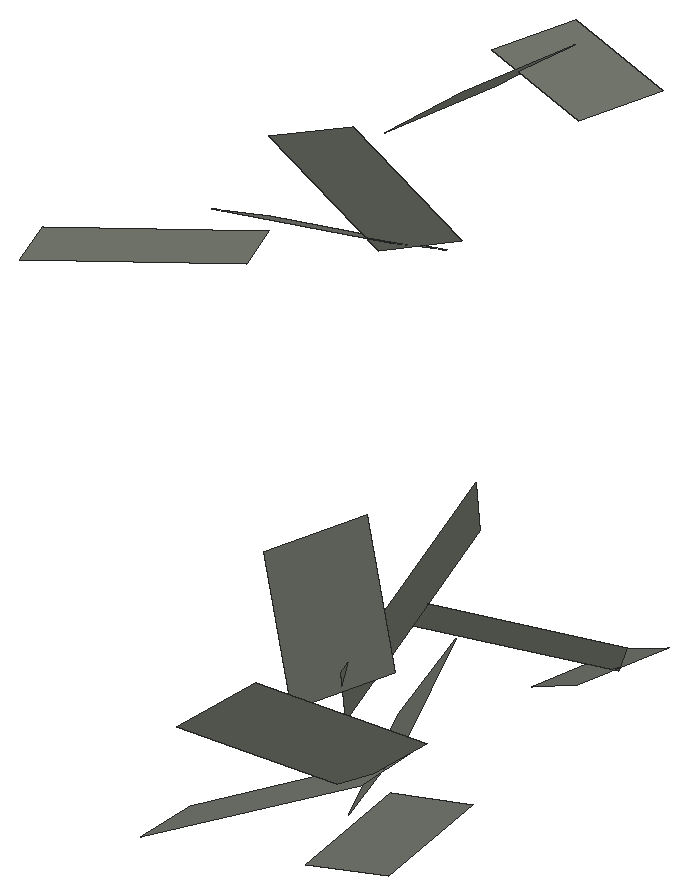
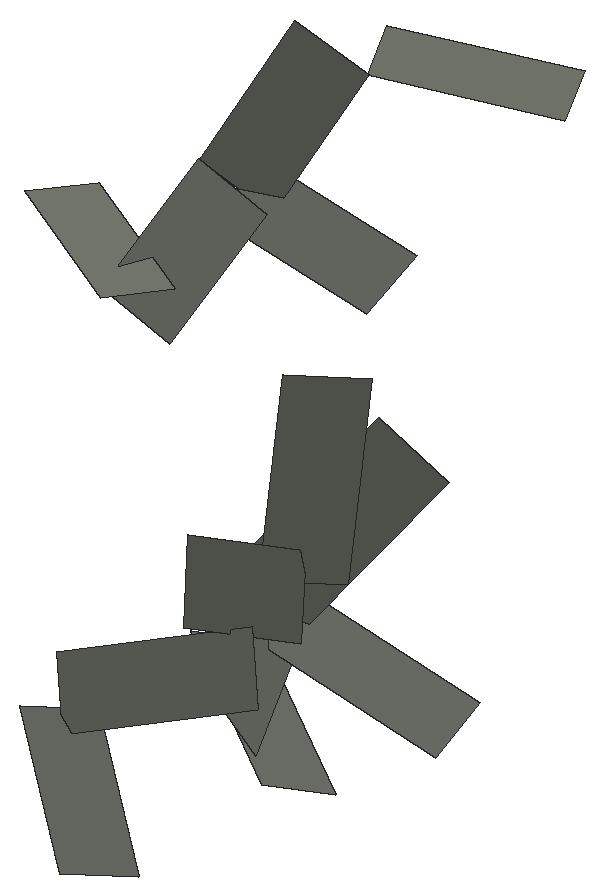
# SketchUp Ruby script. Lengths in inches.
U = 1.inch
M = Sketchup.active_model
def pt(a) = Geom::Point3d.new(a.map { |v| v * U })
def face(e, loops, mat)
  f = e.add_face(loops[0].map { |a| pt(a) })
  loops[1..].each { |l| e.add_face(l.map { |a| pt(a) }).erase! }
  f.material = f.back_material = mat if mat
  f
end
# faces: each face lists its corners as indices into pts; further lists are holes
def faces(e, pts, list, mat = nil) = list.each { |f| face(e, (f[0].is_a?(Array) ? f : [f]).map { |l| l.map { |i| pts[i] } }, mat) }
# xy, xz, yz: faces in a plane at the given z, y or x. An outline is a flat list of corners, or four numbers for a rectangle; further outlines are holes
def ring(l) = l.size == 4 ? [[l[0], l[1]], [l[2], l[1]], [l[2], l[3]], [l[0], l[3]]] : l.each_slice(2).to_a
def flat(e, list, mat, &to3) = list.each { |f| face(e, (f[0].is_a?(Array) ? f : [f]).map { |l| ring(l).map { |u, v| to3.(u, v) } }, mat) }
def xy(e, z, list, mat = nil) = flat(e, list, mat) { |x, y| [x, y, z] }
def xz(e, y, list, mat = nil) = flat(e, list, mat) { |x, z| [x, y, z] }
def yz(e, x, list, mat = nil) = flat(e, list, mat) { |y, z| [x, y, z] }
def lines(e, pts, list) = list.each { |a, b| e.add_line(pt(pts[a]), pt(pts[b])) }
# prism: a flat outline (further loops are holes) pulled along v
def prism(e, loops, v, mat = nil)
  f = face(e, loops, mat); d = Geom::Vector3d.new(v.map { |x| x * U })
  f.pushpull(f.normal.samedirection?(d) ? d.length : -d.length)
end
def box(e, o, s, mat = nil) = prism(e, [[o, [o[0] + s[0], o[1], o[2]], [o[0] + s[0], o[1] + s[1], o[2]], [o[0], o[1] + s[1], o[2]]]], [0, 0, s[2]], mat)
def at(x, y, z, deg = 0) = Geom::Transformation.translation(pt([x, y, z])) * Geom::Transformation.rotation(ORIGIN, Z_AXIS, deg.degrees)
def axes(o, x, y, z) = Geom::Transformation.new([*x, 0, *y, 0, *z, 0, *pt(o).to_a, 1])
def part(name) = M.definitions.add(name)
# library, detail: a bought-in or finely detailed component or shape, given as its bounding box
def library(name, o, s) = part(name).tap { |d| box(d.entities, o, s) }
def detail(e, o, s) = box(e.add_group.entities, o, s)
def put(e, d, t, mat = nil) = e.add_instance(d, t).tap { |i| i.material = mat if mat }
def group(e, t, mat = nil) = e.add_group.tap { |g| g.transformation = t; g.material = mat if mat }.entities
root = M.entities
M.materials.add("viburnumbladsadfasdfad0w122").color = [125, 129, 119]
c1 = part("Component\#315")
p = [[0.25,0,0],[2.05,0.01,0.35],[1.81,4.2,1.66],[0,4.19,1.3125]]
faces(c1.entities,p,[[0,1,2,3]],"viburnumbladsadfasdfad0w122")
c2 = part("viburnumblad2")
put(c2.entities,c1,axes([-19.23,-4.49,-32.18],[83.35428,0,0],[0,79.38502,0],[0,0,83.35428]))
put(root,c2,axes([2192.125,265.73,30.04],[-0.00355,0.00962,-0.00319],[-0.00963,-0.00512,-0.00451],[-0.00533,0.00188,0.0087]))
put(root,c2,axes([2192.16,269.91,28.65],[0.00165,0.00828,-0.00613],[-0.01063,-0.00165,-0.00484],[-0.00434,0.00735,0.00651]))
put(root,c2,axes([2192.3,268.57,18.41],[-0.00076,0.01192,-0.00361],[-0.00919,-0.00341,-0.00868],[-0.0089,0.00223,0.00792]))
put(root,c2,axes([2190.14,272.26,29.11],[0.01,0.00241,0.00568],[0.00061,0.01041,-0.00507],[-0.00589,0.00485,0.00722]))
put(root,c2,axes([2190.53,270.39,18.3],[0.00591,-0.00596,0.00904],[0.00359,0.01104,0.00474],[-0.01042,0.00047,0.00632]))
put(root,c2,axes([2191.57,269.16,17.3],[0.0076,0.00349,0.00917],[-0.0018,0.01107,-0.00252],[-0.00973,0.00035,0.00724]))
put(root,c2,axes([2191.49,270.57,19.52],[-0.00484,-0.0109,-0.00393],[0.00466,-0.0057,0.0098],[-0.01055,0.00253,0.0057]))
put(root,c2,axes([2193.53,274.67,18.95],[-0.00463,0.00496,-0.0092],[-0.00796,-0.0082,-0.00042],[-0.00678,0.00624,0.00678]))
put(root,c2,axes([2192.88,268.62,16.77],[0.00505,0.01138,0.0041],[-0.00637,0.00552,-0.00732],[-0.00911,0.00107,0.00791]))
put(root,c2,axes([2192.54,274.53,17.91],[0.00707,0.00889,0.00124],[-0.00553,0.00556,-0.00832],[-0.00707,0.00455,0.00775]))
put(root,c2,axes([2192.88,269.74,18.95],[-0.0076,-0.00349,-0.00917],[-0.00045,-0.01161,0.00442],[-0.00992,0.00325,0.00636]))
put(root,c2,axes([2193.14,270.71,28.69],[-0.01044,-0.00252,-0.00593],[-0.00181,-0.00803,0.006],[-0.00557,0.00722,0.00577]))
put(root,c2,axes([2193.09,273.92,29.67],[0.00555,0.00919,-0.00035],[-0.00852,0.00498,-0.00446],[-0.00353,0.00247,0.00881]))
